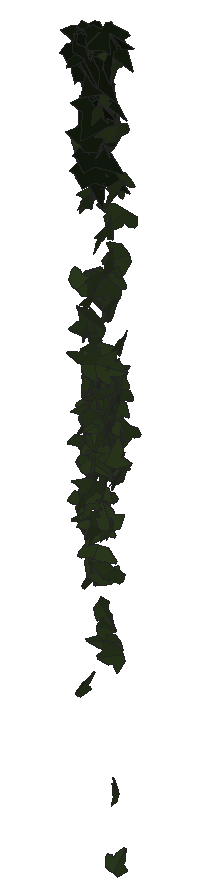
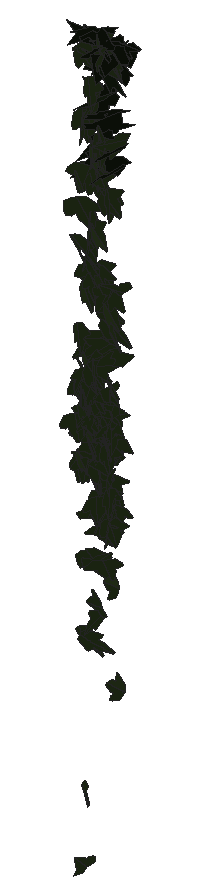
# SketchUp Ruby script. Lengths in inches.
U = 1.inch
M = Sketchup.active_model
def pt(a) = Geom::Point3d.new(a.map { |v| v * U })
def face(e, loops, mat)
  f = e.add_face(loops[0].map { |a| pt(a) })
  loops[1..].each { |l| e.add_face(l.map { |a| pt(a) }).erase! }
  f.material = f.back_material = mat if mat
  f
end
# faces: each face lists its corners as indices into pts; further lists are holes
def faces(e, pts, list, mat = nil) = list.each { |f| face(e, (f[0].is_a?(Array) ? f : [f]).map { |l| l.map { |i| pts[i] } }, mat) }
# xy, xz, yz: faces in a plane at the given z, y or x. An outline is a flat list of corners, or four numbers for a rectangle; further outlines are holes
def ring(l) = l.size == 4 ? [[l[0], l[1]], [l[2], l[1]], [l[2], l[3]], [l[0], l[3]]] : l.each_slice(2).to_a
def flat(e, list, mat, &to3) = list.each { |f| face(e, (f[0].is_a?(Array) ? f : [f]).map { |l| ring(l).map { |u, v| to3.(u, v) } }, mat) }
def xy(e, z, list, mat = nil) = flat(e, list, mat) { |x, y| [x, y, z] }
def xz(e, y, list, mat = nil) = flat(e, list, mat) { |x, z| [x, y, z] }
def yz(e, x, list, mat = nil) = flat(e, list, mat) { |y, z| [x, y, z] }
def lines(e, pts, list) = list.each { |a, b| e.add_line(pt(pts[a]), pt(pts[b])) }
# prism: a flat outline (further loops are holes) pulled along v
def prism(e, loops, v, mat = nil)
  f = face(e, loops, mat); d = Geom::Vector3d.new(v.map { |x| x * U })
  f.pushpull(f.normal.samedirection?(d) ? d.length : -d.length)
end
def box(e, o, s, mat = nil) = prism(e, [[o, [o[0] + s[0], o[1], o[2]], [o[0] + s[0], o[1] + s[1], o[2]], [o[0], o[1] + s[1], o[2]]]], [0, 0, s[2]], mat)
def at(x, y, z, deg = 0) = Geom::Transformation.translation(pt([x, y, z])) * Geom::Transformation.rotation(ORIGIN, Z_AXIS, deg.degrees)
def axes(o, x, y, z) = Geom::Transformation.new([*x, 0, *y, 0, *z, 0, *pt(o).to_a, 1])
def part(name) = M.definitions.add(name)
# library, detail: a bought-in or finely detailed component or shape, given as its bounding box
def library(name, o, s) = part(name).tap { |d| box(d.entities, o, s) }
def detail(e, o, s) = box(e.add_group.entities, o, s)
def put(e, d, t, mat = nil) = e.add_instance(d, t).tap { |i| i.material = mat if mat }
def group(e, t, mat = nil) = e.add_group.tap { |g| g.transformation = t; g.material = mat if mat }.entities
root = M.entities
M.materials.add("1026 AP 7946 SUNNY SIDE UP").color = [254, 231, 186]
M.materials.add("efeu1").color = [18, 25, 13]
M.materials.add("efeu2").color = [43, 57, 29]
c1 = part("ivyleaf_10")
p = [[0,0.5,-0.03],[-0.0625,2.02,-0.43],[-0.19,2.01,-0.46],[-0.54,1.05,-0.29],[-0.52,0.625,-0.18],[-0.83,0.76,-0.28],
  [-1.16,0.64,-0.33],[-1.15,0.33,-0.24],[-0.77,-0.39,0.02],[-0.3,-0.51,0.16],[0.04,-0.48,0.23],[-0.02,2.01,-0.4375],
  [-0.06,2.01,-0.43],[0.04,-0.49,0.23],[0.67,-0.49,0.14],[1.38,0.36,-0.2],[1.375,0.51,-0.24],[0.81,0.65,-0.19],
  [0.62,0.59,-0.15],[0.6,1.09,-0.28],[0.5,1.23,-0.31]]
faces(c1.entities,p,[[0,1,2,3,4,5,6,7,8,9,10],[11,12,0,13,14,15,16,17,18,19,20]],"efeu2")
c2 = part("ivyleaf_9")
p = [[1.54,2.16,1.25],[1.36,2.04,1.19],[-0.21,0.99,0.68],[-0.71,1.11,0.82],[-0.85,0.86,0.67],[-0.8,0.17,0.21],
  [-0.9,-0.01,0.1],[-0.67,-0.16,-0.02],[-0.08,-0.08,-0.05],[-0.03,-0.6,-0.4],[0.65,-0.88,-0.66],[0.83,-0.6,-0.49],
  [1.29,-0.42,-0.43],[1.8125,-0.07,-0.26],[1.21,0.44,0.15]]
faces(c2.entities,p,[[0,1,2,3,4,5,6,7,8,9,10,11,12,13,14]],"efeu1")
put(root,c1,axes([103.92,212.92,257.87],[-0.02385,-0.19968,-0.04275],[0.0443,0.03803,-0.2045],[0.31725,-0.02032,0.02534]),"1026 AP 7946 SUNNY SIDE UP")
put(root,c1,axes([103.84,212.91,261.44],[0.1794,-0.14419,0.14524],[0.13145,-0.11462,-0.19004],[0.28955,0.14137,-0.00371]),"1026 AP 7946 SUNNY SIDE UP")
put(root,c1,axes([103.97,212.8,267.6],[0.26007,-0.19847,-0.04543],[-0.0459,0.03162,-0.26596],[0.31599,0.16794,-0.00124]),"1026 AP 7946 SUNNY SIDE UP")
put(root,c1,axes([103.97,212.96,267.54],[-0.11767,-0.20375,0.13722],[0.02072,-0.1437,-0.21777],[0.3832,-0.05479,0.05391]),"1026 AP 7946 SUNNY SIDE UP")
put(root,c1,axes([103.97,212.76,259.21],[-0.01451,-0.20058,-0.09899],[0.01673,0.09452,-0.20621],[0.34854,-0.01289,0.00578]),"1026 AP 7946 SUNNY SIDE UP")
put(root,c2,axes([104.02,212.98,267.35],[-0.24675,0.11676,-0.16509],[0.18462,-0.111,-0.20159],[-0.25227,-0.19544,0.01395]),"1026 AP 7946 SUNNY SIDE UP")
put(root,c1,axes([104,212.79,257.125],[-0.12714,-0.1959,0.02852],[-0.00559,-0.02967,-0.21835],[0.31129,-0.08055,0.00773]),"1026 AP 7946 SUNNY SIDE UP")
put(root,c1,axes([103.99,212.86,261.9375],[0.04662,-0.21847,0.0637],[-0.00123,-0.06371,-0.22731],[0.35755,0.02827,-0.00909]),"1026 AP 7946 SUNNY SIDE UP")
put(root,c1,axes([104,212.88,258.8],[-0.05417,-0.20209,-0.03639],[0.00728,0.03387,-0.21099],[0.32219,-0.03474,-0.00135]),"1026 AP 7946 SUNNY SIDE UP")
put(root,c1,axes([104.23,212.56,261.41],[-0.17107,0.02965,0.21875],[-0.33533,0.00765,-0.11371],[-0.03205,-0.23831,0.02215]),"1026 AP 7946 SUNNY SIDE UP")
put(root,c1,axes([103.98,212.69,255.7],[0.10364,-0.1376,0.16508],[-0.07896,0.15368,0.15736],[-0.32354,-0.08158,0.01448]),"1026 AP 7946 SUNNY SIDE UP")
put(root,c2,axes([103.91,212.52,267.68],[-0.00921,-0.04367,-0.27136],[-0.07448,0.25921,-0.04171],[0.41279,0.04579,-0.01358]),"1026 AP 7946 SUNNY SIDE UP")
put(root,c1,axes([103.93,212.72,257.51],[0.32366,-0.0021,0.01328],[0.01989,-0.01922,-0.21126],[0.00517,0.20534,-0.01842]),"1026 AP 7946 SUNNY SIDE UP")
put(root,c1,axes([103.98,212.6,257.63],[0.03336,-0.16866,-0.12498],[0.04798,0.12222,-0.17017],[0.32225,-0.00074,0.03828]),"1026 AP 7946 SUNNY SIDE UP")
put(root,c1,axes([104.03,212.74,259.53],[-0.13106,-0.18547,0.05118],[0.00512,-0.05664,-0.20816],[0.3023,-0.07945,0.02572]),"1026 AP 7946 SUNNY SIDE UP")
put(root,c1,axes([103.88,212.64,262.27],[0.16687,0.08441,-0.20356],[0.16849,0.17083,0.13514],[0.29364,-0.14599,0.03813]),"1026 AP 7946 SUNNY SIDE UP")
put(root,c1,axes([103.98,212.54,253.35],[0.0606,-0.13754,0.15517],[-0.03738,0.15001,0.1475],[-0.31945,-0.04364,0.01218]),"1026 AP 7946 SUNNY SIDE UP")
put(root,c2,axes([104.09,212.8,267.77],[-0.34569,-0.1271,0.00216],[0.01362,-0.02059,-0.26074],[0.19944,-0.2189,0.02155]),"1026 AP 7946 SUNNY SIDE UP")
put(root,c1,axes([104.04,212.93,259.11],[0.13143,-0.19156,-0.03723],[-0.02101,0.03242,-0.21512],[0.30549,0.08464,0.00122]),"1026 AP 7946 SUNNY SIDE UP")
put(root,c2,axes([104,212.85,267.78],[0.33511,0.12137,-0.09259],[-0.15238,-0.01083,-0.24997],[-0.18297,0.23131,0.0386]),"1026 AP 7946 SUNNY SIDE UP")
put(root,c1,axes([104.04,212.76,259.4],[-0.31848,0.06894,-0.00567],[-0.00121,-0.02049,-0.2196],[-0.10879,-0.20159,0.01905]),"1026 AP 7946 SUNNY SIDE UP")
put(root,c1,axes([104.05,212.75,260.21],[0.21691,-0.17092,0.01237],[-0.00491,-0.01916,-0.2259],[0.26949,0.13723,-0.01407]),"1026 AP 7946 SUNNY SIDE UP")
put(root,c1,axes([104.1,212.79,264.35],[-0.03382,-0.21131,0.1144],[-0.01444,-0.11189,-0.21946],[0.37596,-0.0233,0.00186]),"1026 AP 7946 SUNNY SIDE UP")
put(root,c1,axes([104.01,212.9,259.33],[0.00314,0.21211,-0.03562],[-0.00302,-0.03576,-0.21873],[-0.33822,0.00229,0.00162]),"1026 AP 7946 SUNNY SIDE UP")
put(root,c1,axes([104.09,212.7,256.99],[0.02953,-0.12218,-0.17493],[-0.00222,0.16972,-0.12549],[0.32804,0.01215,0.01489]),"1026 AP 7946 SUNNY SIDE UP")
put(root,c1,axes([103.98,212.87,258.13],[0.04559,-0.13836,0.1528],[0.14676,-0.12477,-0.13871],[0.28419,0.08663,0.04712]),"1026 AP 7946 SUNNY SIDE UP")
put(root,c1,axes([104.1,212.66,264.33],[-0.01226,-0.21611,-0.10654],[0.00947,0.10203,-0.22218],[0.37577,-0.00962,0.00212]),"1026 AP 7946 SUNNY SIDE UP")
put(root,c1,axes([104.04,212.61,258.9],[-0.29294,-0.07813,-0.05064],[0.09314,-0.01754,-0.20451],[0.11084,-0.19176,0.03802]),"1026 AP 7946 SUNNY SIDE UP")
put(root,c1,axes([104.01,212.82,262.23],[-0.34217,0.007,-0.07603],[0.11227,-0.04216,-0.22115],[-0.03156,-0.2259,0.03755]),"1026 AP 7946 SUNNY SIDE UP")
put(root,c1,axes([104.05,212.91,256.3],[0.25543,0.14993,-0.0653],[-0.05548,-0.05621,-0.22741],[-0.2504,0.1654,-0.01622]),"1026 AP 7946 SUNNY SIDE UP")
put(root,c2,axes([103.92,212.875,265.47],[0.05882,-0.23607,-0.05615],[0.0185,0.0555,-0.24506],[0.38005,0.03384,0.02062]),"1026 AP 7946 SUNNY SIDE UP")
put(root,c1,axes([104.04,212.77,260.12],[0.09219,0.20084,-0.05444],[-0.00958,-0.0544,-0.21565],[-0.32687,0.05824,-0.00903]),"1026 AP 7946 SUNNY SIDE UP")
put(root,c1,axes([103.91,212.79,259.83],[-0.06834,0.01137,-0.21861],[0.20677,-0.16879,-0.03804],[-0.26261,-0.13586,0.02693]),"1026 AP 7946 SUNNY SIDE UP")
put(root,c1,axes([104.1,212.92,260.66],[-0.02339,-0.05839,0.22924],[0.05787,-0.22106,-0.05843],[0.3576,0.03195,0.02445]),"1026 AP 7946 SUNNY SIDE UP")
put(root,c1,axes([104.2,212.63,257.97],[-0.20844,-0.14098,0.08011],[-0.06223,-0.07016,-0.19892],[0.24602,-0.13719,0.01755]),"1026 AP 7946 SUNNY SIDE UP")
put(root,c1,axes([104.17,212.8,257.79],[0.25027,0.07513,-0.10667],[-0.13639,-0.05902,-0.18109],[-0.14859,0.18072,-0.01344]),"1026 AP 7946 SUNNY SIDE UP")
put(root,c1,axes([104.17,212.81,258.79],[-0.09488,-0.17229,0.11115],[-0.00089,-0.11339,-0.18586],[0.32046,-0.05132,0.03239]),"1026 AP 7946 SUNNY SIDE UP")
put(root,c1,axes([103.99,212.48,265.5],[0.10629,-0.01059,-0.27374],[0.20974,0.23846,0.02657],[0.36163,-0.1352,0.06504]),"1026 AP 7946 SUNNY SIDE UP")
put(root,c1,axes([104.13,212.59,260.68],[-0.32557,-0.08972,0.02273],[0.01981,0.02747,0.23171],[-0.14412,0.20646,-0.01949]),"1026 AP 7946 SUNNY SIDE UP")
put(root,c2,axes([104,212.74,267.58],[0.04325,-0.25458,0.02807],[0.00062,-0.02882,-0.26394],[0.40283,0.02738,-0.00261]),"1026 AP 7946 SUNNY SIDE UP")
put(root,c1,axes([104.14,212.81,256.98],[0.27657,0.11608,-0.06501],[-0.06463,-0.05293,-0.21637],[-0.19796,0.17945,-0.02018]),"1026 AP 7946 SUNNY SIDE UP")
put(root,c1,axes([104.15,212.76,259.65],[0.29917,0.0742,-0.05106],[-0.05987,-0.03914,-0.20939],[-0.1273,0.19279,-0.02152]),"1026 AP 7946 SUNNY SIDE UP")
put(root,c1,axes([104.42,212.51,261.61],[-0.03981,0.01189,-0.24873],[-0.2983,0.14959,0.02895],[0.23575,0.19129,-0.00537]),"1026 AP 7946 SUNNY SIDE UP")
put(root,c1,axes([104.1875,212.86,259.4],[0.32271,0.0259,-0.04327],[-0.06539,-0.00714,-0.21314],[-0.04215,0.2094,-0.00067]),"1026 AP 7946 SUNNY SIDE UP")
put(root,c1,axes([104.25,212.83,259.81],[-0.07658,-0.18941,0.09509],[-0.02413,-0.0924,-0.20188],[0.33118,-0.05053,0.00728]),"1026 AP 7946 SUNNY SIDE UP")
put(root,c2,axes([104.08,212.875,267.68],[-0.06941,-0.24184,-0.08153],[0.02975,0.07558,-0.25277],[0.39834,-0.04779,0.00467]),"1026 AP 7946 SUNNY SIDE UP")
put(root,c1,axes([104.27,212.93,258.34],[-0.04182,-0.12913,0.16171],[-0.05309,-0.15405,-0.13672],[0.31606,-0.04297,-0.00157]),"1026 AP 7946 SUNNY SIDE UP")
put(root,c1,axes([104.21,212.8,267.8125],[0.0614,-0.24223,0.0827],[0.02227,-0.08042,-0.25323],[0.40132,0.04152,0.0014]),"1026 AP 7946 SUNNY SIDE UP")
put(root,c1,axes([104.15,212.91,259.26],[0.24116,-0.14487,0.03126],[0.06055,-0.00434,-0.21607],[0.225,0.15644,0.02465]),"1026 AP 7946 SUNNY SIDE UP")
put(root,c1,axes([104.23,212.89,259.27],[0.14238,-0.19004,0.00012],[-0.00905,-0.00407,-0.21677],[0.29869,0.09046,-0.00663]),"1026 AP 7946 SUNNY SIDE UP")
put(root,c2,axes([104.09,212.75,264.875],[0.01904,-0.24274,-0.02013],[0.00042,0.0182,-0.25027],[0.38274,0.01206,0.00128]),"1026 AP 7946 SUNNY SIDE UP")
put(root,c2,axes([104.24,212.85,266.19],[-0.23539,-0.19404,0.06331],[-0.01935,-0.06886,-0.25081],[0.31999,-0.14691,0.0314]),"1026 AP 7946 SUNNY SIDE UP")
put(root,c2,axes([104.02,212.92,266.67],[0.17447,-0.21358,-0.07268],[0.03848,0.08838,-0.2396],[0.35099,0.09648,0.0624]),"1026 AP 7946 SUNNY SIDE UP")
put(root,c2,axes([104.41,212.57,265.6875],[-0.34246,-0.14761,0.08811],[0.09305,0.06617,0.27061],[-0.2523,0.22476,-0.0198]),"1026 AP 7946 SUNNY SIDE UP")
put(root,c1,axes([104.25,212.92,257.59],[-0.18179,-0.16723,0.01591],[0.04847,-0.04067,-0.20368],[0.25973,-0.10946,0.04915]),"1026 AP 7946 SUNNY SIDE UP")
put(root,c1,axes([104.11,212.54,258.62],[-0.04008,-0.10547,-0.19688],[0.22495,0.13649,-0.09677],[0.25814,-0.13532,0.05376]),"1026 AP 7946 SUNNY SIDE UP")
put(root,c1,axes([104.35,212.76,258.14],[0.05734,-0.11012,-0.18145],[-0.09624,0.16452,-0.11848],[0.31125,0.07116,-0.00321]),"1026 AP 7946 SUNNY SIDE UP")
put(root,c1,axes([104.24,212.98,267.67],[0.39594,0.03951,-0.02471],[-0.0436,0.02127,-0.26117],[-0.05838,0.25207,0.02744]),"1026 AP 7946 SUNNY SIDE UP")
put(root,c2,axes([104.28,212.82,266.93],[-0.18741,-0.15784,0.16265],[-0.03698,-0.17006,-0.19334],[0.3501,-0.10246,0.06665]),"1026 AP 7946 SUNNY SIDE UP")
put(root,c1,axes([104.34,212.85,264.71],[-0.09427,-0.21899,0.0782],[-0.01501,-0.07729,-0.2341],[0.36478,-0.05977,0.01057]),"1026 AP 7946 SUNNY SIDE UP")
put(root,c1,axes([104.32,212.73,265.52],[-0.02063,-0.24278,-0.06918],[0.01155,0.06546,-0.25007],[0.39534,-0.01458,0.00369]),"1026 AP 7946 SUNNY SIDE UP")
put(root,c1,axes([104.52,212.875,258.6],[0.04108,0.01201,-0.21279],[-0.32208,-0.02834,-0.02855],[-0.04663,0.20632,0.0097]),"1026 AP 7946 SUNNY SIDE UP")
put(root,c1,axes([104.52,212.86,254.46],[0.12192,-0.01024,-0.19648],[-0.29802,0.02077,-0.08044],[0.03633,0.20478,-0.00046]),"1026 AP 7946 SUNNY SIDE UP")
put(root,c1,axes([104.34,213.01,266.89],[0.00511,-0.23946,-0.07472],[0.00557,0.07121,-0.24625],[0.39276,0.00211,0.00446]),"1026 AP 7946 SUNNY SIDE UP")
put(root,c1,axes([104.36,212.67,262.6],[-0.01448,-0.22527,0.08228],[-0.01483,-0.0808,-0.23266],[0.3762,-0.01186,-0.00601]),"1026 AP 7946 SUNNY SIDE UP")
put(root,c2,axes([104.07,212.625,267.29],[-0.08655,-0.08601,-0.25182],[0.3561,0.1045,-0.08999],[0.19654,-0.22721,0.05215]),"1026 AP 7946 SUNNY SIDE UP")
put(root,c1,axes([104.34,212.83,263.55],[0.0831,-0.21788,0.09215],[0.02046,-0.0901,-0.23135],[0.37052,0.05384,-0.00789]),"1026 AP 7946 SUNNY SIDE UP")
put(root,c1,axes([104.375,212.92,260.49],[-0.03896,-0.20865,0.10007],[-0.00562,-0.09853,-0.2169],[0.36264,-0.02394,0.00739]),"1026 AP 7946 SUNNY SIDE UP")
put(root,c1,axes([104.32,212.74,258.59],[-0.01498,-0.15771,0.1523],[0.05984,-0.14778,-0.15978],[0.33557,0.01931,0.03529]),"1026 AP 7946 SUNNY SIDE UP")
put(root,c1,axes([104.29,212.41,260.74],[0.00202,0.05218,0.26313],[-0.00154,0.25513,-0.05226],[-0.40946,-0.0007,0.00149]),"1026 AP 7946 SUNNY SIDE UP")
put(root,c2,axes([104.02,212.95,267.74],[0.28,-0.03526,-0.18771],[0.28896,0.06683,0.17228],[0.03841,-0.2457,0.07222]),"1026 AP 7946 SUNNY SIDE UP")
put(root,c1,axes([104.35,212.86,265.32],[0.07252,-0.2224,0.09921],[0.03794,-0.09462,-0.2345],[0.37998,0.05189,0.00448]),"1026 AP 7946 SUNNY SIDE UP")
put(root,c1,axes([104.34,212.46,257.17],[0.04142,-0.12866,-0.21541],[0.05968,0.20918,-0.1269],[0.38041,-0.01881,0.04336]),"1026 AP 7946 SUNNY SIDE UP")
put(root,c1,axes([104.4,212.76,260.5],[0.04631,-0.19758,-0.12084],[-0.01615,0.11588,-0.20502],[0.36004,0.03061,0.00635]),"1026 AP 7946 SUNNY SIDE UP")
put(root,c1,axes([104.33,212.91,259.46],[0.08239,0.20603,-0.02712],[-0.03383,-0.02283,-0.21859],[-0.32508,0.05459,0.01588]),"1026 AP 7946 SUNNY SIDE UP")
put(root,c1,axes([104.3,212.9,258.01],[0.14752,-0.14402,0.11459],[0.10449,-0.09037,-0.17751],[0.26722,0.11484,0.00616]),"1026 AP 7946 SUNNY SIDE UP")
put(root,c1,axes([104.4,212.66,265.74],[0.18783,-0.21704,-0.05551],[-0.02596,0.05096,-0.25472],[0.35021,0.12019,0.01089]),"1026 AP 7946 SUNNY SIDE UP")
put(root,c1,axes([104.29,212.51,259.7],[-0.05545,-0.18874,-0.1714],[0.16465,0.14062,-0.1876],[0.35851,-0.09377,0.05965]),"1026 AP 7946 SUNNY SIDE UP")
put(root,c1,axes([104.57,212.64,262.53],[-0.29586,0.01197,0.1413],[-0.21502,-0.04234,-0.18978],[0.0243,-0.22892,0.0411]),"1026 AP 7946 SUNNY SIDE UP")
put(root,c1,axes([104.37,212.8,262.52],[-0.12279,-0.21791,-0.0046],[0.07968,-0.01482,-0.23229],[0.33329,-0.07674,0.05384]),"1026 AP 7946 SUNNY SIDE UP")
put(root,c1,axes([104.4375,212.75,264.97],[0.12604,-0.20058,-0.11926],[-0.04293,0.11225,-0.22137],[0.36071,0.08345,0.01532]),"1026 AP 7946 SUNNY SIDE UP")
put(root,c1,axes([104.17,212.51,258.56],[0.16,0.07783,0.18328],[0.23028,0.10038,-0.13127],[-0.19954,0.17825,-0.00453]),"1026 AP 7946 SUNNY SIDE UP")
put(root,c1,axes([104.51,212.69,259.48],[0.24053,0.06043,-0.15352],[-0.21535,-0.05974,-0.16974],[-0.13347,0.20529,-0.00279]),"1026 AP 7946 SUNNY SIDE UP")
put(root,c2,axes([104.21,212.53,265.09],[0.038,-0.09258,-0.24919],[0.06557,0.24063,-0.08938],[0.40115,-0.03056,0.03822]),"1026 AP 7946 SUNNY SIDE UP")
put(root,c2,axes([104.26,212.46,265.49],[0.06603,-0.09757,-0.23417],[-0.0214,0.22875,-0.10266],[0.38757,0.02925,0.03423]),"1026 AP 7946 SUNNY SIDE UP")
put(root,c1,axes([104.37,212.69,259.35],[0.32938,0.06687,-0.02509],[-0.02692,-0.02733,-0.22569],[-0.10883,0.20915,-0.0201]),"1026 AP 7946 SUNNY SIDE UP")
put(root,c2,axes([104.15,212.71,266.4],[0.10187,-0.10575,0.22707],[0.1609,-0.19604,-0.12868],[0.35005,0.12089,-0.00693]),"1026 AP 7946 SUNNY SIDE UP")
put(root,c1,axes([104.49,212.73,265.32],[0.09625,-0.06985,-0.24109],[-0.06905,0.23378,-0.08249],[0.37715,0.06062,0.04642]),"1026 AP 7946 SUNNY SIDE UP")
put(root,c1,axes([104.47,212.76,262.61],[-0.34356,-0.07551,0.03244],[-0.01329,-0.06963,-0.2297],[0.12822,-0.20955,0.06312]),"1026 AP 7946 SUNNY SIDE UP")
put(root,c1,axes([104.42,212.96,260.08],[-0.33388,0.02925,-0.02585],[0.03359,-0.02873,-0.21943],[-0.05065,-0.2119,0.02489]),"1026 AP 7946 SUNNY SIDE UP")
put(root,c1,axes([104.41,212.65,254.86],[0.00892,0.09817,0.18463],[-0.04521,0.17733,-0.0984],[-0.31734,-0.0225,0.01921]),"1026 AP 7946 SUNNY SIDE UP")
put(root,c1,axes([104.41,212.92,258.89],[0.17127,-0.18084,0.01362],[0.0161,-0.01046,-0.21752],[0.28478,0.10935,0.00411]),"1026 AP 7946 SUNNY SIDE UP")
put(root,c1,axes([104.25,212.64,260.9375],[0.17732,0.13089,0.14786],[0.15519,0.10333,-0.17729],[-0.26207,0.14975,-0.00494]),"1026 AP 7946 SUNNY SIDE UP")
put(root,c1,axes([104.51,212.66,255.98],[0.16763,0.14737,0.0982],[-0.10289,-0.06906,0.18662],[0.25531,-0.12459,0.01073]),"1026 AP 7946 SUNNY SIDE UP")
put(root,c1,axes([104.54,212.91,251.12],[0.02729,-0.06073,-0.201],[-0.10882,0.18212,-0.06379],[0.30176,0.07117,-0.00483]),"1026 AP 7946 SUNNY SIDE UP")
put(root,c1,axes([104.38,212.88,259.85],[0.28432,-0.11518,0.03589],[0.05507,-0.01102,-0.22072],[0.18134,0.18394,0.01075]),"1026 AP 7946 SUNNY SIDE UP")
put(root,c1,axes([104.52,212.65,259.79],[0.17732,-0.17797,-0.06632],[-0.06926,0.04699,-0.21644],[0.28885,0.12051,-0.01119]),"1026 AP 7946 SUNNY SIDE UP")
put(root,c1,axes([104.5,212.84,260.33],[-0.29602,-0.11299,0.02641],[0.01781,-0.06775,-0.21693],[0.18153,-0.1776,0.06435]),"1026 AP 7946 SUNNY SIDE UP")
put(root,c1,axes([104.43,212.5625,266.47],[-0.02677,-0.17038,-0.22686],[0.10285,0.21101,-0.17293],[0.4243,-0.06189,0.02761]),"1026 AP 7946 SUNNY SIDE UP")
put(root,c1,axes([104.46,212.81,263.76],[0.07301,-0.22015,-0.09819],[0.05011,0.10065,-0.22588],[0.37309,0.02956,0.04955]),"1026 AP 7946 SUNNY SIDE UP")
put(root,c1,axes([104.4375,212.89,260.1],[0.25738,-0.13603,0.03127],[0.03318,-0.02329,-0.21934],[0.21689,0.16498,-0.00355]),"1026 AP 7946 SUNNY SIDE UP")
put(root,c1,axes([104.625,212.66,256.17],[-0.24963,-0.08818,0.12197],[-0.14265,-0.07981,-0.18623],[0.18393,-0.18158,0.02111]),"1026 AP 7946 SUNNY SIDE UP")
put(root,c1,axes([104.37,212.875,258.52],[0.30161,0.07432,0.04611],[0.07687,-0.0041,-0.21084],[-0.11229,0.19683,-0.02049]),"1026 AP 7946 SUNNY SIDE UP")
put(root,c1,axes([104.52,212.74,259.45],[-0.11872,-0.18747,0.07724],[0.00927,-0.08317,-0.20569],[0.31797,-0.06757,0.03484]),"1026 AP 7946 SUNNY SIDE UP")
put(root,c2,axes([104.32,212.8125,267.76],[-0.17095,-0.02742,-0.24563],[0.37567,-0.03542,-0.10831],[-0.03321,-0.2595,0.03917]),"1026 AP 7946 SUNNY SIDE UP")
put(root,c1,axes([104.47,212.92,258.375],[-0.23309,-0.14092,-0.02548],[0.07272,-0.01466,-0.20626],[0.21266,-0.14944,0.0426]),"1026 AP 7946 SUNNY SIDE UP")
put(root,c1,axes([104.27,212.78,255.21],[0.11899,-0.01316,0.19953],[0.28123,-0.0763,-0.07775],[0.11898,0.19351,-0.01577]),"1026 AP 7946 SUNNY SIDE UP")
put(root,c1,axes([104.53,212.73,257.15],[0.14687,0.1951,0.01149],[-0.02269,-0.00422,0.22252],[0.30635,-0.09385,0.01097]),"1026 AP 7946 SUNNY SIDE UP")
put(root,c1,axes([104.46,212.95,259.4],[0.01174,0.18211,-0.11014],[-0.00464,-0.10791,-0.18839],[-0.33284,0.00793,-0.00126]),"1026 AP 7946 SUNNY SIDE UP")
put(root,c1,axes([104.55,212.7,259.35],[0.09405,-0.1937,-0.0648],[-0.02217,0.06032,-0.20845],[0.31893,0.06131,0.00462]),"1026 AP 7946 SUNNY SIDE UP")
put(root,c1,axes([104.51,212.9,264.84],[-0.37355,0.02328,-0.03434],[0.04756,-0.03202,-0.24432],[-0.04298,-0.23776,0.02811]),"1026 AP 7946 SUNNY SIDE UP")
put(root,c1,axes([104.55,212.68,257.16],[0.18066,-0.17237,-0.02777],[-0.03317,0.01713,-0.21315],[0.27208,0.11654,-0.00755]),"1026 AP 7946 SUNNY SIDE UP")
put(root,c1,axes([104.56,212.9,259.63],[-0.01919,-0.21484,0.01197],[0.00007,-0.01286,-0.22175],[0.33841,-0.01218,0.00072]),"1026 AP 7946 SUNNY SIDE UP")
put(root,c1,axes([104.54,212.88,259.84],[0.10051,-0.2057,-0.0231],[0.00933,0.02406,-0.22138],[0.32504,0.06292,0.0135]),"1026 AP 7946 SUNNY SIDE UP")
put(root,c1,axes([104.53,212.92,262.87],[0.27184,-0.15699,-0.00102],[-0.01295,-0.00892,-0.2403],[0.24651,0.17265,-0.01149]),"1026 AP 7946 SUNNY SIDE UP")
put(root,c1,axes([104.51,212.92,249.4375],[0.09112,0.12763,-0.15313],[0.07479,0.14199,0.14482],[0.29974,-0.07422,0.01042]),"1026 AP 7946 SUNNY SIDE UP")
put(root,c2,axes([104.35,212.78,268],[0.02298,-0.20971,-0.15452],[0.09665,0.14757,-0.20717],[0.3926,-0.02405,0.06004]),"1026 AP 7946 SUNNY SIDE UP")
put(root,c1,axes([104.46,212.89,259.44],[-0.27586,0.06197,-0.10545],[0.13573,-0.06114,-0.19026],[-0.13097,-0.19388,0.02493]),"1026 AP 7946 SUNNY SIDE UP")
put(root,c1,axes([104.5625,212.97,260.38],[-0.02119,0.19041,0.10291],[-0.0646,0.09489,-0.19358],[-0.33108,-0.0307,0.03118]),"1026 AP 7946 SUNNY SIDE UP")
put(root,c1,axes([104.62,212.86,260.04],[-0.25936,-0.13535,0.02835],[-0.01697,-0.03129,-0.21928],[0.21675,-0.1644,0.01675]),"1026 AP 7946 SUNNY SIDE UP")
put(root,c1,axes([104.71,212.88,264.04],[-0.32308,-0.06748,0.11237],[-0.14091,-0.07282,-0.21998],[0.145,-0.22112,0.03659]),"1026 AP 7946 SUNNY SIDE UP")
put(root,c1,axes([104.56,212.68,263.05],[0.04054,-0.16601,-0.16709],[0.05306,0.16321,-0.16659],[0.36003,-0.00536,0.04337]),"1026 AP 7946 SUNNY SIDE UP")
put(root,c1,axes([104.55,212.93,266.04],[0.10381,-0.22016,-0.10238],[0.05088,0.10892,-0.22868],[0.37558,0.0461,0.05928]),"1026 AP 7946 SUNNY SIDE UP")
put(root,c1,axes([104.61,212.88,267.5],[-0.08505,-0.21127,0.14083],[0.01787,-0.14293,-0.22183],[0.3963,-0.03889,0.04023]),"1026 AP 7946 SUNNY SIDE UP")
put(root,c1,axes([104.6,212.74,259.43],[0.00278,-0.20203,-0.10145],[0.03776,0.09694,-0.20629],[0.35058,-0.00884,0.02302]),"1026 AP 7946 SUNNY SIDE UP")
put(root,c1,axes([104.62,212.94,258.53],[0.04158,-0.20315,0.03214],[-0.00144,-0.03273,-0.21118],[0.32346,0.02597,-0.00507]),"1026 AP 7946 SUNNY SIDE UP")
put(root,c1,axes([104.625,212.65,262.09],[0.22572,-0.17977,-0.01924],[-0.02633,0.00921,-0.23683],[0.28281,0.14434,-0.00669]),"1026 AP 7946 SUNNY SIDE UP")
put(root,c1,axes([104.61,212.89,258.4],[-0.15605,-0.17578,-0.05143],[0.0498,0.03825,-0.20754],[0.28254,-0.10383,0.00817]),"1026 AP 7946 SUNNY SIDE UP")
put(root,c1,axes([104.57,212.55,259.26],[-0.05457,-0.16451,-0.1512],[0.12638,0.12792,-0.16762],[0.32174,-0.07815,0.04019]),"1026 AP 7946 SUNNY SIDE UP")
put(root,c1,axes([104.78,212.8,263.17],[0.23096,-0.12534,-0.15521],[-0.20751,0.07474,-0.1971],[0.22666,0.19614,-0.0223]),"1026 AP 7946 SUNNY SIDE UP")
put(root,c1,axes([104.79,212.625,254.39],[0.1938,-0.09215,-0.17098],[-0.22157,0.08725,-0.1577],[0.19894,0.18695,-0.00908]),"1026 AP 7946 SUNNY SIDE UP")
put(root,c1,axes([104.59,212.58,259.45],[-0.08507,0.19897,-0.04619],[0.00834,-0.04617,-0.21257],[-0.32099,-0.05393,0.00672]),"1026 AP 7946 SUNNY SIDE UP")
put(root,c1,axes([104.67,212.73,262.12],[0.02135,-0.22846,0.00475],[-0.00525,-0.00612,-0.23578],[0.35932,0.01348,-0.00372]),"1026 AP 7946 SUNNY SIDE UP")
put(root,c1,axes([104.61,212.86,259.8],[0.31801,-0.06849,0.00526],[-0.0017,-0.02025,-0.21917],[0.10802,0.20131,-0.01893]),"1026 AP 7946 SUNNY SIDE UP")
put(root,c1,axes([104.69,212.74,265.96],[-0.14291,-0.23674,0.00547],[0.00446,-0.00822,-0.26123],[0.37237,-0.09076,0.00523]),"1026 AP 7946 SUNNY SIDE UP")
put(root,c1,axes([104.625,212.79,260.7],[0.07175,-0.18794,0.11183],[0.06514,-0.10245,-0.19931],[0.33585,0.06002,0.01477]),"1026 AP 7946 SUNNY SIDE UP")
put(root,c1,axes([104.66,212.88,260.11],[0.10141,-0.2014,-0.05405],[0.0381,0.06065,-0.21349],[0.32457,0.05581,0.04195]),"1026 AP 7946 SUNNY SIDE UP")
put(root,c1,axes([104.72,212.88,261.24],[0.02076,-0.21968,-0.06028],[0.00061,0.05739,-0.22635],[0.35696,0.01268,0.00389]),"1026 AP 7946 SUNNY SIDE UP")
put(root,c1,axes([104.73,212.77,258.32],[0.06553,-0.20261,-0.0188],[-0.01754,0.01515,-0.21285],[0.31923,0.04242,-0.00784]),"1026 AP 7946 SUNNY SIDE UP")
put(root,c1,axes([104.59,212.6,258.69],[0.36077,0.00555,-0.05518],[0.08235,0.03219,0.23458],[0.01993,-0.2334,0.02965]),"1026 AP 7946 SUNNY SIDE UP")
put(root,c1,axes([104.72,212.8,264.69],[0.03473,-0.2028,0.13003],[0.0102,-0.12736,-0.21081],[0.37643,0.02216,-0.00629]),"1026 AP 7946 SUNNY SIDE UP")
put(root,c1,axes([104.65,212.4,260.83],[0.00211,0.1192,0.24231],[0.01898,0.23426,-0.12136],[-0.41324,0.01136,-0.00434]),"1026 AP 7946 SUNNY SIDE UP")
put(root,c1,axes([104.77,212.92,259.25],[-0.25375,-0.13346,0.02676],[-0.01181,-0.03267,-0.21492],[0.21369,-0.16028,0.0199]),"1026 AP 7946 SUNNY SIDE UP")
put(root,c1,axes([104.64,212.92,260.41],[-0.10026,0.05774,-0.20536],[0.0694,-0.20033,-0.07537],[-0.31937,-0.06166,0.04809]),"1026 AP 7946 SUNNY SIDE UP")
